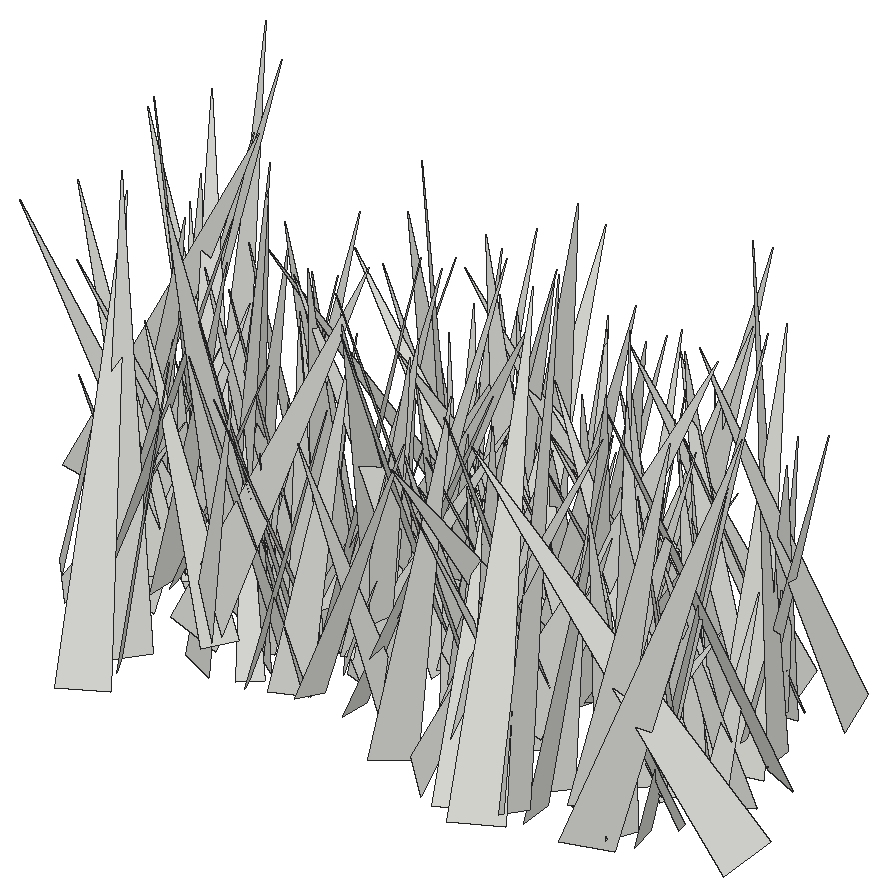
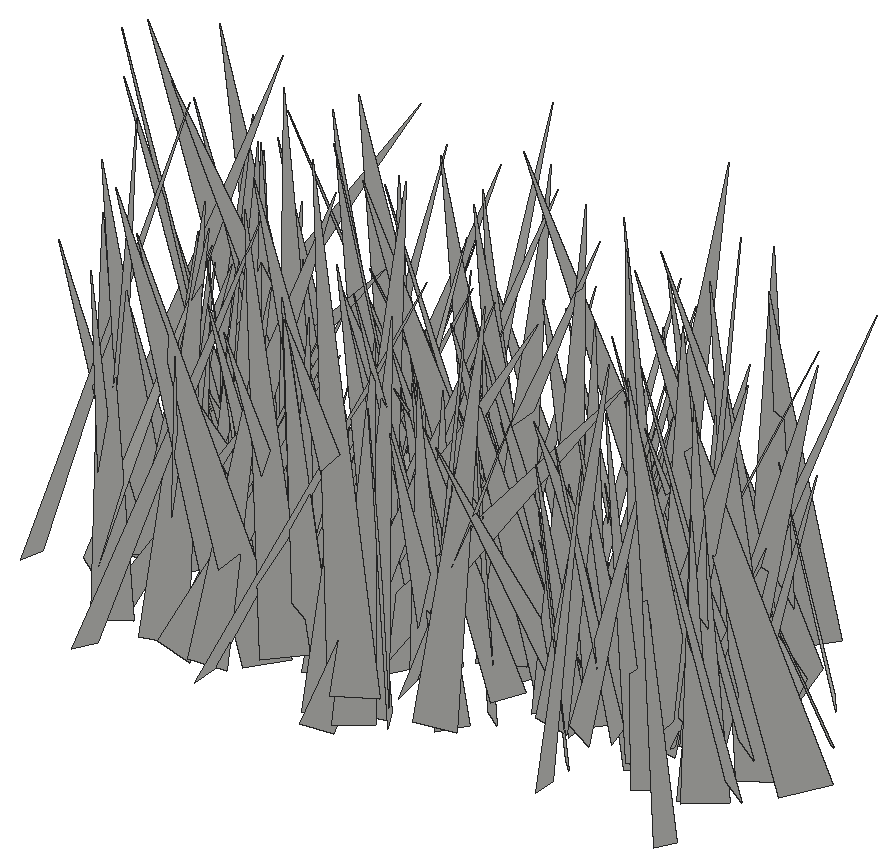
# SketchUp Ruby script. Lengths in inches.
U = 1.inch
M = Sketchup.active_model
def pt(a) = Geom::Point3d.new(a.map { |v| v * U })
def face(e, loops, mat)
  f = e.add_face(loops[0].map { |a| pt(a) })
  loops[1..].each { |l| e.add_face(l.map { |a| pt(a) }).erase! }
  f.material = f.back_material = mat if mat
  f
end
# faces: each face lists its corners as indices into pts; further lists are holes
def faces(e, pts, list, mat = nil) = list.each { |f| face(e, (f[0].is_a?(Array) ? f : [f]).map { |l| l.map { |i| pts[i] } }, mat) }
# xy, xz, yz: faces in a plane at the given z, y or x. An outline is a flat list of corners, or four numbers for a rectangle; further outlines are holes
def ring(l) = l.size == 4 ? [[l[0], l[1]], [l[2], l[1]], [l[2], l[3]], [l[0], l[3]]] : l.each_slice(2).to_a
def flat(e, list, mat, &to3) = list.each { |f| face(e, (f[0].is_a?(Array) ? f : [f]).map { |l| ring(l).map { |u, v| to3.(u, v) } }, mat) }
def xy(e, z, list, mat = nil) = flat(e, list, mat) { |x, y| [x, y, z] }
def xz(e, y, list, mat = nil) = flat(e, list, mat) { |x, z| [x, y, z] }
def yz(e, x, list, mat = nil) = flat(e, list, mat) { |y, z| [x, y, z] }
def lines(e, pts, list) = list.each { |a, b| e.add_line(pt(pts[a]), pt(pts[b])) }
# prism: a flat outline (further loops are holes) pulled along v
def prism(e, loops, v, mat = nil)
  f = face(e, loops, mat); d = Geom::Vector3d.new(v.map { |x| x * U })
  f.pushpull(f.normal.samedirection?(d) ? d.length : -d.length)
end
def box(e, o, s, mat = nil) = prism(e, [[o, [o[0] + s[0], o[1], o[2]], [o[0] + s[0], o[1] + s[1], o[2]], [o[0], o[1] + s[1], o[2]]]], [0, 0, s[2]], mat)
def at(x, y, z, deg = 0) = Geom::Transformation.translation(pt([x, y, z])) * Geom::Transformation.rotation(ORIGIN, Z_AXIS, deg.degrees)
def axes(o, x, y, z) = Geom::Transformation.new([*x, 0, *y, 0, *z, 0, *pt(o).to_a, 1])
def part(name) = M.definitions.add(name)
# library, detail: a bought-in or finely detailed component or shape, given as its bounding box
def library(name, o, s) = part(name).tap { |d| box(d.entities, o, s) }
def detail(e, o, s) = box(e.add_group.entities, o, s)
def put(e, d, t, mat = nil) = e.add_instance(d, t).tap { |i| i.material = mat if mat }
def group(e, t, mat = nil) = e.add_group.tap { |g| g.transformation = t; g.material = mat if mat }.entities
root = M.entities
c1 = part("fur_instance\#9")
p = [[0.8125,0,1.79],[0.67,-0.02,1.48],[0,-0.11,0],[0,0.11,0]]
faces(c1.entities,p,[[0,1,2,3]])
put(root,c1,axes([115.82,140.54,-28.22],[-5.29033,5.65073,1.03717],[5.57546,5.38985,-0.92613],[1.38587,-0.11308,7.68509]))
put(root,c1,axes([131.42,139.93,-27.1],[-6.0602,5.67803,0.65626],[5.53411,6.06799,-1.39639],[1.4298,0.57987,8.18634]))
put(root,c1,axes([133.57,142.85,-27.1],[4.4224,-5.22883,1.99199],[-5.58659,-4.26873,1.19762],[-0.31423,2.30295,6.7427]))
put(root,c1,axes([137.84,144.91,-28.22],[-7.44265,2.94787,0.75024],[2.95668,6.54484,3.6151],[-0.71474,-3.62229,7.14241]))
put(root,c1,axes([125.74,143.01,-28.22],[5.12868,-4.19399,1.94705],[-4.5125,-5.17419,0.74098],[-1.00889,1.82269,6.58361]))
put(root,c1,axes([126.9375,142.61,-28.22],[5.08074,5.57509,0.64514],[5.46993,-4.72427,-2.25231],[1.25607,-1.97773,7.19879]))
put(root,c1,axes([122.61,142.9375,-27.1],[4.92372,-1.23429,0.65682],[-1.32256,-4.89156,0.72207],[-0.45359,0.86432,5.02445]))
put(root,c1,axes([117.61,143.8,-28.22],[-0.80392,-5.00028,1.94874],[-5.12712,1.2977,1.21465],[1.58527,1.66129,4.91668]))
put(root,c1,axes([133.63,142.47,-28.22],[6.06814,-4.77445,2.10475],[-5.2154,-5.64781,2.22478],[-0.15808,3.05854,7.39379]))
put(root,c1,axes([115.74,142.39,-28.22],[4.42151,2.80893,1.55928],[2.73673,-4.68252,0.67492],[-1.68278,-0.23477,5.19464]))
put(root,c1,axes([128.92,141.76,-28.22],[-2.44616,4.11048,0.29857],[4.09909,2.46258,-0.31948],[0.42742,-0.0923,4.7726]))
put(root,c1,axes([128.84,145.5,-27.1],[-3.83157,-3.11067,0.41222],[-2.87249,3.73899,1.51524],[1.26294,-0.9332,4.69694]))
put(root,c1,axes([115.6,142.85,-28.22],[5.91163,-3.56463,4.13587],[-4.286,-6.80601,0.26026],[-3.38262,2.39395,6.89828]))
put(root,c1,axes([123.98,145.26,-28.22],[-5.24413,-0.63684,1.6828],[-0.10679,5.28634,1.66778],[1.7961,-1.54509,5.01248]))
put(root,c1,axes([120.3,146.12,-27.1],[-2.61623,-5.06997,0.16776],[-4.93297,2.58676,1.24576],[1.18261,-0.42604,5.56752]))
put(root,c1,axes([131.2,143.05,-28.22],[6.35559,1.23086,1.81432],[1.1106,-6.60444,0.5901],[-1.89033,0.25813,6.44673]))
put(root,c1,axes([118.55,143.7,-27.1],[-3.73959,3.61146,1.09906],[3.77498,3.58144,1.07604],[0.00944,-1.53809,5.08619]))
put(root,c1,axes([114.375,142.4375,-28.22],[7.43833,2.19546,1.23858],[2.06036,-7.51855,0.95355],[-1.45225,0.57818,7.69672]))
put(root,c1,axes([120.96,144.51,-28.22],[-2.70694,-4.99144,1.16007],[-5.08628,2.45713,-1.29614],[-0.62448,1.62351,5.52829]))
put(root,c1,axes([131.83,141.22,-27.1],[-7.99125,0.08509,2.25297],[-0.74491,7.73167,-2.93422],[2.12796,3.02611,7.43355]))
put(root,c1,axes([135.36,144.99,-27.1],[-3.25628,-4.53556,1.56998],[-4.60157,3.48952,0.53691],[1.36443,0.94415,5.55755]))
put(root,c1,axes([117.53,143.7,-27.1],[1.82991,-7.19945,3.13467],[-7.38413,-0.48301,3.20126],[2.67073,3.59742,6.70317]))
put(root,c1,axes([119.28,144.3,-28.22],[5.27684,1.71083,0.85913],[1.8324,-5.24307,-0.81398],[-0.55438,-1.04563,5.4872]))
put(root,c1,axes([120.6,145.05,-28.22],[-4.07714,-4.72232,1.18622],[-4.85623,4.056,-0.54439],[0.3528,1.25658,6.21506]))
put(root,c1,axes([132.38,143.8,-28.22],[2.74298,6.25055,1.8619],[6.47418,-2.36552,-1.59662],[0.78801,-2.32269,6.63657]))
put(root,c1,axes([129.05,146.65,-27.1],[-2.89154,-5.8907,0.51675],[-5.81601,2.937,0.93617],[1.06836,0.04534,6.49499]))
put(root,c1,axes([136.35,143.625,-27.1],[-4.35257,-4.39527,0.35538],[-3.69396,3.36161,-3.66659],[-2.40819,2.78761,4.98191]))
put(root,c1,axes([124.13,147.74,-27.1],[-3.49524,-7.20934,0.56433],[-6.86604,3.50524,2.25399],[2.26947,-0.49846,7.68835]))
put(root,c1,axes([113.61,145.07,-27.1],[5.71322,-0.96407,0.62556],[-0.92485,-5.73993,-0.39936],[-0.68221,-0.29224,5.7802]))
put(root,c1,axes([117.31,146.64,-27.1],[6.25935,-4.83068,2.00086],[-4.50057,-6.56633,-1.77386],[-2.66155,-0.25726,7.70509]))
put(root,c1,axes([127.67,145.03,-27.1],[-4.9951,-5.23204,0.99068],[-5.30492,4.77148,-1.54841],[-0.46216,1.77916,7.06595]))
put(root,c1,axes([119.0625,145.21,-28.22],[-1.65671,-3.63214,1.3485],[-3.6613,1.94738,0.7471],[1.26719,0.87797,3.92161]))
put(root,c1,axes([132.0625,145.66,-27.1],[2.34766,-4.1804,1.05082],[-4.25289,-2.44131,-0.21062],[-0.70205,0.80976,4.78987]))
put(root,c1,axes([130.82,144.6,-28.22],[-3.54773,2.23846,2.32232],[2.39169,4.14191,-0.33862],[2.16418,-0.90784,4.1812]))
put(root,c1,axes([126.87,146.09,-27.1],[1.30695,-5.86281,0.96642],[-5.89292,-1.15208,0.98022],[0.76158,1.14664,5.9262]))
put(root,c1,axes([127.87,149.27,-28.22],[6.60243,-3.6292,1.16999],[-2.40466,-5.77841,-4.35427],[-2.95933,-3.40161,6.14845]))
put(root,c1,axes([120.83,144.19,-28.22],[3.9195,-3.82723,2.46639],[-4.43668,-3.94163,0.93419],[-1.02305,2.43088,5.39791]))
put(root,c1,axes([122.37,145.98,-28.22],[0.32033,-6.88611,1.90206],[-6.92731,0.16595,1.76741],[1.74605,1.92169,6.66313]))
put(root,c1,axes([111.55,144.95,-28.22],[3.27011,3.05252,0.13659],[2.8317,-2.95233,-1.81533],[1.14804,-1.41282,4.08853]))
put(root,c1,axes([111.87,144.43,-27.1],[3.13745,2.7412,0.96065],[2.81213,-3.22064,0.00574],[-0.7273,-0.62763,4.16626]))
put(root,c1,axes([119.43,144.07,-28.22],[-2.46678,3.0111,0.36551],[3.02886,2.4705,0.08915],[0.1623,-0.33942,3.8915]))
put(root,c1,axes([129.21,146.8,-27.1],[-4.78281,-0.5343,0.54387],[-0.29464,4.48183,1.81189],[0.70318,-1.75621,4.45846]))
put(root,c1,axes([114.99,145.56,-27.1],[6.44965,-0.53992,1.19924],[-0.48241,-6.55498,-0.35669],[-1.22351,-0.26161,6.46237]))
put(root,c1,axes([120.39,145.75,-28.22],[-2.89225,-3.68575,0.79235],[-3.76683,2.78458,-0.79678],[-0.15371,1.11313,4.61682]))
put(root,c1,axes([122.49,145.73,-27.1],[4.00541,-4.88826,1.49079],[-5.10449,-3.91872,0.86522],[-0.24835,1.7057,6.26017]))
put(root,c1,axes([113.32,146.625,-27.1],[-1.78915,-3.44674,0.35763],[-3.41457,1.82215,0.479],[0.59044,0.09337,3.85378]))
put(root,c1,axes([136.88,147.69,-27.1],[-3.06964,-6.81398,0.3454],[-6.81954,3.05272,-0.38339],[-0.20825,0.47214,7.46364]))
put(root,c1,axes([115.08,147.53,-28.22],[-7.55604,-1.18176,1.01335],[-0.88861,7.39753,2.00103],[1.27821,-1.84315,7.38147]))
put(root,c1,axes([126.48,144.35,-28.22],[4.76351,-2.22786,1.63166],[-2.67424,-4.53288,1.61806],[-0.68857,2.19233,5.00362]))
put(root,c1,axes([117.125,147.14,-27.1],[-5.82237,-2.50943,0.01956],[-2.48564,5.77362,0.82736],[0.34528,-0.75212,6.28591]))
put(root,c1,axes([122.29,145.02,-27.1],[3.35941,2.47012,0.56366],[2.52325,-3.34641,-0.37364],[-0.22894,-0.63632,4.15301]))
put(root,c1,axes([115.23,146.33,-27.1],[1.42662,-4.11071,0.89066],[-4.20545,-1.41051,0.22612],[-0.07357,0.91596,4.34535]))
put(root,c1,axes([134.03,143.63,-28.22],[-7.61718,0.0241,1.98426],[-0.51537,7.57673,-2.07045],[1.91631,2.1335,7.33043]))
put(root,c1,axes([122.96,144.67,-28.22],[6.06997,0.80019,0.53139],[0.73411,-6.05703,0.73529],[-0.61948,0.66277,6.07817]))
put(root,c1,axes([120.125,145.82,-27.1],[-0.91503,4.79321,2.31879],[5.31141,0.98733,0.05504],[0.37492,-2.28894,4.87946]))
put(root,c1,axes([121.08,148.78,-27.1],[6.38764,-4.10189,0.26345],[-3.90919,-6.21298,-1.95294],[-1.27011,-1.50671,7.33577]))
put(root,c1,axes([128.78,146.22,-28.22],[1.11597,-3.30458,1.27259],[-3.40234,-1.37051,-0.57526],[-0.98175,0.99326,3.44016]))
put(root,c1,axes([131.78,145.19,-28.22],[0.48143,3.7055,0.846],[3.27794,0.02687,-1.98307],[1.92393,-0.97302,3.16701]))
put(root,c1,axes([126.15,147.21,-28.22],[0.3349,-5.08877,0.86463],[-5.08924,-0.4702,-0.79617],[-0.86188,0.79915,5.03725]))
put(root,c1,axes([113.18,144.39,-27.1],[4.04294,1.47662,0.10602],[1.40514,-3.92456,1.07725],[-0.46609,0.97696,4.16717]))
put(root,c1,axes([122.45,145.25,-27.1],[3.25743,4.86298,0.41292],[4.6269,-2.91916,-2.12138],[1.55271,-1.50328,5.4552]))
put(root,c1,axes([122.65,147.09,-27.1],[1.67883,-4.20753,0.33675],[-4.18563,-1.61266,0.71764],[0.54516,0.57551,4.47289]))
put(root,c1,axes([124.76,147.01,-27.1],[-6.87538,0.87455,0.95023],[1.06547,6.75006,1.49673],[0.72976,-1.61573,6.76724]))
put(root,c1,axes([115.11,145.99,-27.1],[4.62251,0.92588,0.22465],[0.9419,-4.60847,-0.38752],[-0.14333,-0.42437,4.69837]))
put(root,c1,axes([114.61,145.97,-27.1],[0.94645,-5.69848,3.07489],[-6.04954,-1.88624,-1.63358],[-2.30884,2.60631,5.54074]))
put(root,c1,axes([134.625,143.89,-28.22],[7.20277,3.49638,1.97973],[3.12762,-7.42996,1.74287],[-2.5223,0.77133,7.81454]))
put(root,c1,axes([129.4375,147.79,-27.1],[6.44633,-3.37101,0.63256],[-3.2949,-6.46051,-0.8512],[-0.95262,-0.46602,7.22457]))
put(root,c1,axes([132.48,146.13,-28.22],[4.6761,-4.10232,2.76945],[-4.45315,-5.14998,-0.1096],[-2.16064,1.73593,6.21956]))
put(root,c1,axes([117.5,145.6,-27.1],[3.62939,6.32437,2.66269],[6.74766,-3.83695,-0.08396],[-1.24771,-2.35377,7.2913]))
put(root,c1,axes([133.3,147.05,-27.1],[-1.38247,-3.90181,0.99129],[-3.91317,1.54858,0.63797],[0.94545,0.70412,4.09003]))
put(root,c1,axes([125.81,149.38,-27.1],[-3.26721,-5.06008,0.08616],[-4.54982,2.98181,2.58736],[2.21606,-1.33826,5.43917]))
put(root,c1,axes([119.08,144.82,-28.22],[1.88548,3.67223,0.79609],[3.49899,-2.04056,1.12569],[-1.36969,-0.15771,3.97154]))
put(root,c1,axes([128.86,146.5,-27.1],[3.23817,-2.36152,0.30304],[-2.37388,-3.16317,0.7165],[0.18248,0.75624,3.94324]))
put(root,c1,axes([126.04,147.32,-27.1],[3.30583,-2.31707,0.74955],[-2.21165,-3.38553,-0.71128],[-1.01942,-0.16893,3.97384]))
put(root,c1,axes([128.5,145.55,-27.1],[2.77972,-6.83526,2.99642],[-7.05556,-1.36449,3.4327],[2.43278,3.85274,6.53179]))
put(root,c1,axes([134.58,144.75,-27.1],[1.50713,3.43781,0.3216],[3.3001,-1.53741,0.96906],[-1.01552,0.10596,3.62641]))
put(root,c1,axes([133.91,145.32,-27.1],[-3.45696,-5.56122,4.74392],[-6.59951,4.63089,0.61955],[3.14299,3.60698,6.51874]))
put(root,c1,axes([123.89,144.91,-27.1],[3.6487,6.36792,1.23917],[6.47764,-3.65398,-0.29593],[-0.35515,-1.22351,7.3332]))
put(root,c1,axes([119.24,148.45,-28.22],[7.0973,-2.99001,1.53723],[-2.6894,-7.20395,-1.59536],[-2.01752,-0.91535,7.53436]))
put(root,c1,axes([133.84,146.83,-28.22],[-5.92654,3.46188,1.28835],[3.68281,5.72588,1.55549],[0.28525,-1.99951,6.68498]))
put(root,c1,axes([135.77,147.28,-28.22],[0.22156,-4.52657,1.23949],[-4.53883,-0.5223,-1.09609],[-1.19379,1.1457,4.39744]))
put(root,c1,axes([111.91,147.98,-28.22],[1.15039,-7.47242,1.55869],[-7.41634,-0.72104,2.01691],[1.80677,1.79806,7.28646]))
put(root,c1,axes([118.25,146.42,-28.22],[-4.07706,-2.14403,0.24298],[-2.12817,3.90987,-1.20919],[-0.35608,1.18084,4.44491]))
put(root,c1,axes([125.69,145.88,-27.1],[2.40724,3.27999,1.19788],[3.2967,-2.61439,0.53362],[-1.15108,-0.62824,4.03341]))
put(root,c1,axes([113.86,145.75,-28.22],[0.82135,5.31818,1.14764],[5.3338,-0.55827,-1.23031],[1.07271,-1.29616,5.2387]))
put(root,c1,axes([119.33,147.19,-27.1],[3.22787,2.03353,0.24614],[1.96333,-2.94045,-1.45397],[0.58408,-1.35405,3.52709]))
put(root,c1,axes([113.44,148.88,-28.22],[1.96703,-4.29578,0.10046],[-4.18734,-1.94112,-1.01553],[-0.96439,-0.33368,4.61429]))
put(root,c1,axes([124.96,146.76,-27.1],[2.68991,-2.47286,1.2383],[-2.72716,-2.65872,0.6147],[-0.45937,1.30393,3.60178]))
put(root,c1,axes([121.11,147.38,-28.22],[5.85705,-5.48153,0.51052],[-5.36351,-5.5136,2.33363],[1.24121,2.04104,7.67505]))
put(root,c1,axes([135.15,146.5,-28.22],[-1.54021,3.23682,1.39983],[3.28512,1.87235,-0.71486],[1.28237,-0.90889,3.51258]))
put(root,c1,axes([131.56,148.08,-28.22],[-4.92901,3.2655,3.81824],[4.17297,5.6397,0.56365],[2.798,-2.65855,5.88565]))
put(root,c1,axes([119.26,146.49,-28.22],[-2.16703,-5.16397,2.37315],[-5.48971,1.24499,-2.30381],[-1.47021,2.96275,5.10441]))
put(root,c1,axes([130.63,148.13,-27.1],[1.50872,-3.69838,0.31644],[-3.67115,-1.43625,0.71715],[0.54852,0.55997,3.92937]))
put(root,c1,axes([114.0625,147.78,-28.22],[2.0816,-3.74764,1.04429],[-3.88491,-2.06538,0.3318],[-0.20701,1.076,4.27408]))
put(root,c1,axes([119.02,147.875,-28.22],[2.82941,3.82153,3.56935],[4.50896,-3.83832,0.53527],[-2.64833,-2.45217,4.72474]))
put(root,c1,axes([122.6,145.37,-27.1],[-0.90144,4.87523,0.09791],[4.65666,0.89022,-1.45364],[1.44671,0.1723,4.73998]))
put(root,c1,axes([123.39,148.5,-28.22],[4.68677,-2.0034,0.66372],[-1.95488,-4.73014,-0.47351],[-0.79535,-0.17932,5.07496]))
put(root,c1,axes([120.81,146.01,-27.1],[5.6278,2.51424,1.57514],[2.22036,-5.80941,1.3399],[-1.96786,0.63554,6.01649]))
put(root,c1,axes([127.95,147.63,-27.1],[-0.77592,-4.15559,2.31409],[-4.39268,1.52537,1.26634],[1.82437,1.90534,4.03328]))
put(root,c1,axes([113.79,148.94,-27.1],[-5.15951,-5.90719,2.53837],[-5.9684,5.61072,0.92562],[2.3909,1.25844,7.78837]))
put(root,c1,axes([129.41,147.95,-27.1],[-1.9475,3.70978,1.3462],[3.85912,1.47603,1.51527],[-0.82582,-1.85103,3.9063]))
put(root,c1,axes([134.76,147.77,-28.22],[0.28684,-3.45624,1.82339],[-3.70035,-0.82791,-0.9872],[-1.25608,1.64973,3.32465]))
put(root,c1,axes([123.7,148.13,-28.22],[6.05057,5.41917,1.99571],[5.77348,-5.74186,-1.9125],[-0.1309,-2.76104,7.89425]))
put(root,c1,axes([133.67,149.53,-28.22],[4.64418,-2.47093,1.08294],[-2.19439,-4.71399,-1.3452],[-1.56935,-0.72073,5.0857]))
put(root,c1,axes([128.89,149.39,-28.22],[-2.4025,-2.92839,0.44923],[-2.80853,2.4353,0.85486],[0.94311,-0.20767,3.69008]))
put(root,c1,axes([131.45,149.46,-27.1],[-1.6318,-4.41068,0.10105],[-4.3461,1.58854,-0.8456],[-0.75876,0.38671,4.62621]))
put(root,c1,axes([115.875,146.57,-27.1],[-4.53452,6.13099,1.20513],[6.2123,4.58336,0.05748],[0.66981,-1.00349,7.62546]))
put(root,c1,axes([119.76,147.625,-27.1],[-4.39525,1.44739,0.73649],[1.42922,4.45652,-0.22883],[0.77116,-0.01,4.62177]))
put(root,c1,axes([125.32,146.49,-28.22],[-5.70107,0.73605,0.76728],[0.48907,5.53142,-1.67238],[0.94409,1.57933,5.49974]))
put(root,c1,axes([123.07,149.22,-28.22],[-1.65824,-4.82946,1.36253],[-4.95542,1.80194,0.35604],[0.78993,1.16588,5.09379]))
put(root,c1,axes([133.13,148.66,-28.22],[-4.23654,2.45749,2.21286],[2.8358,4.54981,0.37637],[1.70124,-1.46429,4.88322]))
put(root,c1,axes([120.4,147.13,-28.22],[6.30569,-0.68619,2.05979],[-1.17683,-6.39727,1.4715],[-1.82446,1.75482,6.16987]))
put(root,c1,axes([122.9375,149.11,-28.22],[-1.26744,-3.38882,1.28492],[-3.35573,1.6115,0.94004],[1.36901,0.81271,3.49382]))
put(root,c1,axes([126.78,148.15,-27.1],[0.00954,3.59248,1.3323],[3.47361,-0.5704,1.51319],[-1.6171,-1.20405,3.25826]))
put(root,c1,axes([128.93,149.14,-27.1],[-2.91318,-3.12111,0.33199],[-3.12229,2.8354,-0.74159],[-0.32068,0.74655,4.20452]))
put(root,c1,axes([127.3,148.23,-27.1],[6.46627,-2.11143,1.67342],[-2.36842,-6.52888,0.91405],[-1.28416,1.40953,6.74057]))
put(root,c1,axes([132.09,149.64,-28.22],[-4.86082,-0.82699,0.28427],[-0.77768,4.82218,0.73078],[0.39992,-0.67448,4.87621]))
put(root,c1,axes([109.21,149.13,-27.1],[3.50419,-7.42751,1.71848],[-7.22357,-2.63012,3.36199],[2.43745,2.88357,7.49295]))
put(root,c1,axes([118.5,145.6,-28.22],[-6.46453,1.71895,1.7422],[0.79023,6.12289,-3.109],[2.31637,2.70842,5.92275]))
put(root,c1,axes([133.57,148.49,-28.22],[-3.13424,-4.33981,2.11732],[-4.81159,3.01955,-0.93345],[0.40688,2.2779,5.27125]))
put(root,c1,axes([117.66,148.24,-28.22],[2.7326,-2.75522,2.01665],[-3.2693,-2.85632,0.52755],[-0.98478,1.83723,3.84448]))
put(root,c1,axes([125.54,149.77,-28.22],[3.74176,-6.61768,2.63887],[-6.89022,-4.11933,-0.5604],[-1.81167,1.99888,7.58159]))
put(root,c1,axes([115.83,148.3125,-28.22],[-2.60972,7.0339,1.93347],[7.14895,2.0575,2.16424],[-1.45142,-2.51309,7.18348]))
put(root,c1,axes([127.16,149.38,-28.22],[-6.72983,3.60579,0.05795],[3.45053,6.40273,2.3226],[-1.04828,-2.07339,7.27309]))
put(root,c1,axes([112.75,150.16,-28.22],[2.15592,-3.18911,0.31319],[-3.19535,-2.16794,-0.07942],[-0.24138,0.21478,3.84865]))
put(root,c1,axes([115.16,149.72,-28.22],[0.14432,-5.01914,1.5992],[-4.96199,0.40759,1.72702],[1.76858,1.55311,4.71487]))
put(root,c1,axes([129.51,148.01,-27.1],[4.38555,-0.36882,0.03632],[-0.36139,-4.16033,1.38975],[0.08213,1.3878,4.17584]))
put(root,c1,axes([112.98,152.03,-27.1],[-1.84089,-7.99139,1.4242],[-7.16502,2.28604,3.56596],[3.81486,0.4373,7.3848]))
put(root,c1,axes([131.72,146.2,-28.22],[1.21236,6.8418,0.01969],[6.58716,-1.17263,1.87473],[-1.84929,0.30844,6.6907]))
put(root,c1,axes([118.07,148.84,-28.22],[4.45017,0.43948,1.54669],[0.28501,-4.6951,0.51402],[-1.58245,0.39027,4.44218]))
put(root,c1,axes([112.15,148.28,-27.1],[3.861,5.57007,1.34937],[5.71182,-3.87341,-0.35436],[-0.47072,-1.31331,6.76812]))
put(root,c1,axes([114.56,147.83,-28.22],[-0.8171,5.77252,0.59098],[5.63961,0.64951,1.4532],[-1.36602,-0.77139,5.64605]))
put(root,c1,axes([126.35,151.13,-28.22],[3.47774,-1.50181,0.39234],[-1.2719,-3.30895,-1.39185],[-0.88975,-1.13996,3.5232]))
put(root,c1,axes([119.64,150.22,-27.1],[2.07826,-5.21506,0.82935],[-4.82149,-1.51054,2.58366],[2.15357,1.65083,4.98405]))
put(root,c1,axes([124.36,151.29,-27.1],[-2.66612,-3.28273,0.28859],[-3.19335,2.6653,0.81637],[0.81369,-0.29607,4.14946]))
put(root,c1,axes([112.35,150,-28.22],[3.75494,-4.9741,2.2471],[-5.32599,-3.93562,0.18806],[-1.1937,1.91308,6.22943]))
put(root,c1,axes([120.48,149.95,-28.22],[2.85129,3.39796,1.84964],[3.79237,-2.9092,-0.50161],[-0.76499,-1.75715,4.40731]))
put(root,c1,axes([124.3,147.78,-27.1],[2.11808,6.39246,0.96016],[6.39192,-2.22182,0.69185],[-0.96378,-0.68681,6.6986]))
put(root,c1,axes([129.39,149.99,-27.1],[4.62058,2.87983,1.50344],[3.15499,-4.60106,-0.88304],[-0.77446,-1.56215,5.37246]))
put(root,c1,axes([117.57,150.77,-27.1],[-0.73911,-5.79285,1.55471],[-5.99778,0.70592,-0.22109],[-0.03032,1.57006,5.83563]))
put(root,c1,axes([134.41,148.72,-28.22],[-2.30774,6.81626,2.09214],[7.04491,2.51871,-0.43516],[1.09893,-1.8327,7.18315]))
put(root,c1,axes([136.09,152.3125,-27.1],[-7.13222,-2.21187,1.52983],[-1.72076,7.08542,2.22194],[2.06682,-1.73369,7.12909]))
put(root,c1,axes([123.41,149.07,-27.1],[-6.49961,-2.89491,2.26898],[-3.37847,6.5202,-1.35892],[1.4542,2.20912,6.98418]))
put(root,c1,axes([128.4,148.8,-27.1],[-0.17119,5.69768,1.30234],[5.83131,0.07859,0.42267],[-0.39436,-1.31119,5.68456]))
put(root,c1,axes([133.4,149.9375,-27.1],[-5.24229,2.67543,1.59997],[2.88849,5.34612,0.52444],[1.17239,-1.20849,5.86212]))
put(root,c1,axes([125.35,151.61,-28.22],[-2.19661,-7.3796,0.4517],[-6.30745,1.62463,-4.13089],[-3.85727,1.54587,6.49764]))
put(root,c1,axes([136,148.65,-27.1],[-7.59721,-1.99805,2.32928],[-2.54922,7.5713,-1.81993],[1.70857,2.41215,7.64184]))
put(root,c1,axes([124.16,153.68,-28.22],[6.08199,-2.63161,2.26399],[-1.13407,-5.82276,-3.72169],[-3.281,-2.8656,5.48316]))
put(root,c1,axes([134.52,149.21,-27.1],[5.06172,0.87175,1.3003],[0.68802,-5.19178,0.80241],[-1.40619,0.59773,5.07318]))
put(root,c1,axes([121.03,151.16,-28.22],[4.77577,-2.2799,0.31782],[-2.26651,-4.78515,-0.26858],[-0.40236,-0.10607,5.28524]))
put(root,c1,axes([134.33,151.79,-27.1],[-3.22391,-4.50813,0.36238],[-4.51102,3.23719,0.13952],[0.32445,0.21334,5.54053]))
put(root,c1,axes([113.35,149.11,-27.1],[0.59003,4.76484,1.13067],[4.77949,-0.80843,0.91275],[-1.06703,-0.9864,4.71367]))
put(root,c1,axes([115.65,150.02,-27.1],[4.51759,1.55237,1.02195],[1.60919,-4.61101,-0.10928],[-0.92991,-0.4377,4.77562]))
put(root,c1,axes([114.1,151.03,-27.1],[-0.90647,-5.11686,1.80724],[-5.12934,1.40604,1.40817],[1.7715,1.45288,5.00209]))
put(root,c1,axes([126.54,151.65,-27.1],[1.54796,-4.76639,0.70367],[-4.81569,-1.50748,0.38266],[0.1508,0.78667,4.99682]))
put(root,c1,axes([116.57,150.72,-27.1],[-1.858,-4.3991,1.45242],[-4.62148,1.65138,-0.9103],[-0.32175,1.68364,4.68782]))
put(root,c1,axes([116.97,150.78,-28.22],[2.93725,2.51058,1.33666],[2.80043,-2.8887,-0.72813],[-0.49727,-1.43859,3.79478]))
put(root,c1,axes([119.65,147.94,-27.1],[4.83042,2.64277,1.00625],[2.0268,-4.62442,2.4159],[-1.97202,1.72053,4.9478]))
put(root,c1,axes([123.18,151.05,-27.1],[5.25974,-3.61511,1.15521],[-3.73911,-5.27428,0.51907],[-0.65007,1.0869,6.36116]))
put(root,c1,axes([133.02,152.33,-28.22],[2.32461,-5.72045,0.33614],[-5.68592,-2.25756,0.90225],[0.71192,0.64824,6.10846]))
put(root,c1,axes([130.39,152.7,-28.22],[0.56796,-5.36738,0.34113],[-5.01782,-0.65229,-1.90884],[-1.93561,0.11605,5.04853]))
put(root,c1,axes([126.36,152.44,-27.1],[4.17782,-5.39394,0.17375],[-5.37681,-4.14138,0.71959],[0.46328,0.57738,6.78461]))
put(root,c1,axes([122.23,150.77,-27.1],[-2.98009,3.50221,2.17702],[3.82104,3.35523,-0.16707],[1.55067,-1.53712,4.59549]))
put(root,c1,axes([133.49,151.46,-28.22],[-4.01783,2.35497,0.3103],[2.27352,3.63609,1.84258],[-0.68795,-1.73727,4.27712]))
put(root,c1,axes([134.39,150.64,-27.1],[4.53301,0.32886,1.81446],[0.26511,-4.88148,0.22244],[-1.82486,0.10775,4.53948]))
put(root,c1,axes([131.05,152.38,-28.22],[2.40943,-6.40182,1.38295],[-6.51779,-2.4885,-0.16399],[-0.64358,1.23501,6.83826]))
put(root,c1,axes([114.94,148.22,-27.1],[-7.79963,1.89477,1.60693],[1.33324,7.65978,-2.56065],[2.09639,2.17814,7.60707]))
put(root,c1,axes([127.8,149.4,-27.1],[5.12063,-0.00436,1.95562],[-0.62511,-5.19742,1.62522],[-1.85303,1.74129,4.85588]))
put(root,c1,axes([129.13,152.67,-28.22],[0.8568,-5.86099,0.80486],[-5.91149,-0.87995,-0.11477],[-0.231,0.77949,5.92218]))
put(root,c1,axes([123.46,152.18,-28.22],[1.49133,-6.04191,1.54576],[-6.23212,-1.50337,0.13646],[-0.23383,1.53405,6.22175]))
put(root,c1,axes([128.78,153.17,-28.22],[-7.35388,-1.92649,0.06127],[-1.88282,7.23164,1.39751],[0.41243,-1.33667,7.47248]))
put(root,c1,axes([110.86,150.51,-27.1],[4.61104,6.12434,1.67223],[6.3457,-4.50796,-0.9879],[-0.18966,-1.93296,7.60219]))
put(root,c1,axes([125.81,151.78,-27.1],[2.0151,-5.02328,1.60572],[-5.27188,-1.87389,0.75376],[0.13771,1.76848,5.35965]))
put(root,c1,axes([125.07,148.96,-28.22],[-3.83392,6.10516,1.11787],[5.9137,3.99214,-1.52073],[1.88436,-0.10697,7.04694]))
put(root,c1,axes([116.68,152.23,-28.22],[-4.71927,-1.33587,1.95814],[-1.09743,5.09822,0.83318],[2.10107,-0.33763,4.83341]))
put(root,c1,axes([122.28,151.71,-27.1],[-5.21279,-1.15752,0.50027],[-1.17064,5.23306,-0.0898],[0.46875,0.19648,5.33901]))
put(root,c1,axes([124.6875,152.93,-28.22],[2.32528,-3.90872,0.2043],[-3.90658,-2.33236,-0.15975],[-0.24182,0.09371,4.54527]))
put(root,c1,axes([120.24,152.97,-27.1],[1.37866,-6.43403,1.32521],[-6.55871,-1.42426,-0.09169],[-0.36909,1.27608,6.57944]))
put(root,c1,axes([123.24,153.07,-27.1],[1.49707,-8.01218,1.60299],[-8.01526,-1.12338,1.87068],[1.58751,1.88383,7.93327]))
put(root,c1,axes([132.68,154.04,-28.22],[-7.04471,-1.4589,1.32068],[-0.96261,6.83613,2.41686],[1.71638,-2.15394,6.77607]))
put(root,c1,axes([132.35,150.17,-28.22],[-5.01766,-1.40088,1.70753],[-1.93126,4.83928,-1.7049],[1.07162,2.16194,4.92267]))
put(root,c1,axes([111.68,152.72,-28.22],[4.41728,-0.60705,0.29796],[-0.51929,-4.30631,-1.07505],[-0.43316,-1.02804,4.32726]))
put(root,c1,axes([122.96,149.23,-28.22],[-5.97598,0.81352,1.54005],[0.17172,5.75229,-2.37225],[1.73323,2.235,5.54496]))
put(root,c1,axes([123.46,152.79,-28.22],[4.45698,-3.93649,1.376],[-3.92382,-4.64074,-0.56675],[-1.41173,0.47074,5.91941]))
put(root,c1,axes([129.8125,150.25,-28.22],[7.25129,-2.23194,2.73946],[-2.93898,-7.28136,1.84704],[-1.96177,2.6585,7.35875]))
put(root,c1,axes([122.79,151.95,-28.22],[4.15437,2.45212,1.76514],[2.75663,-4.30471,-0.50784],[-1.23677,-1.35794,4.79727]))
put(root,c1,axes([127.78,151.51,-28.22],[3.27115,-5.93629,2.22387],[-6.24966,-2.60094,2.25],[1.06155,2.98013,6.39355]))
